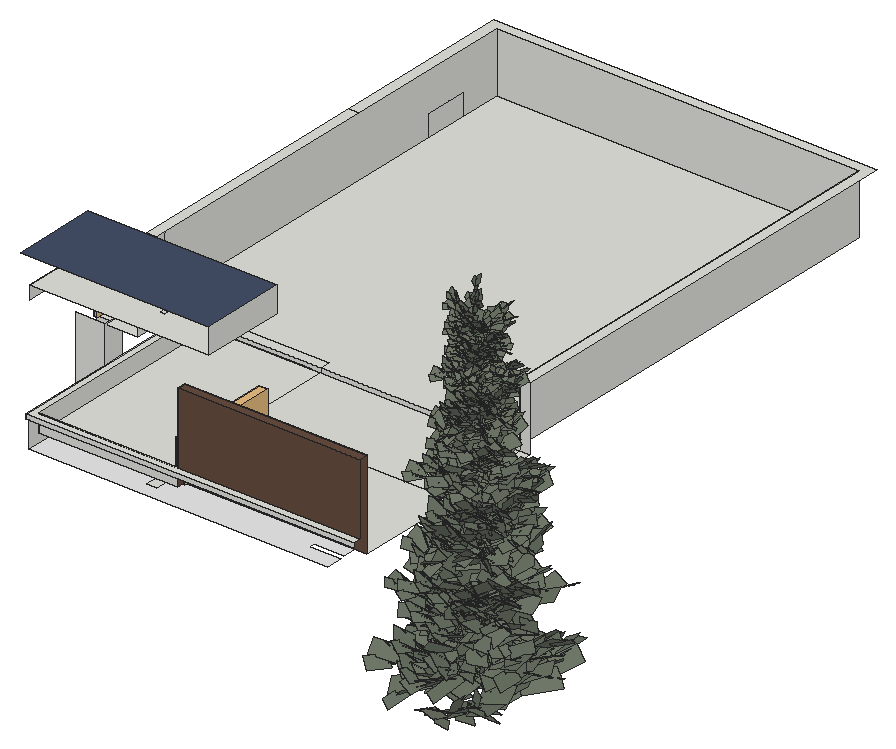
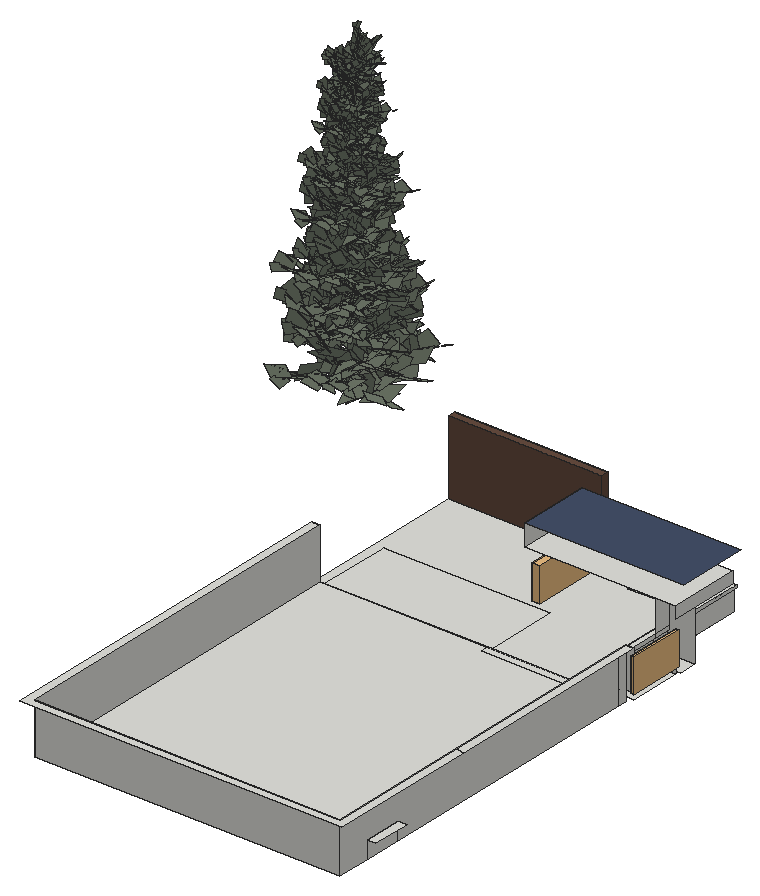
# SketchUp Ruby script. Lengths in inches.
U = 1.inch
M = Sketchup.active_model
def pt(a) = Geom::Point3d.new(a.map { |v| v * U })
def face(e, loops, mat)
  f = e.add_face(loops[0].map { |a| pt(a) })
  loops[1..].each { |l| e.add_face(l.map { |a| pt(a) }).erase! }
  f.material = f.back_material = mat if mat
  f
end
# faces: each face lists its corners as indices into pts; further lists are holes
def faces(e, pts, list, mat = nil) = list.each { |f| face(e, (f[0].is_a?(Array) ? f : [f]).map { |l| l.map { |i| pts[i] } }, mat) }
# xy, xz, yz: faces in a plane at the given z, y or x. An outline is a flat list of corners, or four numbers for a rectangle; further outlines are holes
def ring(l) = l.size == 4 ? [[l[0], l[1]], [l[2], l[1]], [l[2], l[3]], [l[0], l[3]]] : l.each_slice(2).to_a
def flat(e, list, mat, &to3) = list.each { |f| face(e, (f[0].is_a?(Array) ? f : [f]).map { |l| ring(l).map { |u, v| to3.(u, v) } }, mat) }
def xy(e, z, list, mat = nil) = flat(e, list, mat) { |x, y| [x, y, z] }
def xz(e, y, list, mat = nil) = flat(e, list, mat) { |x, z| [x, y, z] }
def yz(e, x, list, mat = nil) = flat(e, list, mat) { |y, z| [x, y, z] }
def lines(e, pts, list) = list.each { |a, b| e.add_line(pt(pts[a]), pt(pts[b])) }
# prism: a flat outline (further loops are holes) pulled along v
def prism(e, loops, v, mat = nil)
  f = face(e, loops, mat); d = Geom::Vector3d.new(v.map { |x| x * U })
  f.pushpull(f.normal.samedirection?(d) ? d.length : -d.length)
end
def box(e, o, s, mat = nil) = prism(e, [[o, [o[0] + s[0], o[1], o[2]], [o[0] + s[0], o[1] + s[1], o[2]], [o[0], o[1] + s[1], o[2]]]], [0, 0, s[2]], mat)
def at(x, y, z, deg = 0) = Geom::Transformation.translation(pt([x, y, z])) * Geom::Transformation.rotation(ORIGIN, Z_AXIS, deg.degrees)
def axes(o, x, y, z) = Geom::Transformation.new([*x, 0, *y, 0, *z, 0, *pt(o).to_a, 1])
def part(name) = M.definitions.add(name)
# library, detail: a bought-in or finely detailed component or shape, given as its bounding box
def library(name, o, s) = part(name).tap { |d| box(d.entities, o, s) }
def detail(e, o, s) = box(e.add_group.entities, o, s)
def put(e, d, t, mat = nil) = e.add_instance(d, t).tap { |i| i.material = mat if mat }
def group(e, t, mat = nil) = e.add_group.tap { |g| g.transformation = t; g.material = mat if mat }.entities
root = M.entities
M.materials.add("Marc_Shoes2").color = [68, 80, 105]
M.materials.add("Teddy_Glasses").color = [103, 77, 64]
M.materials.add("[Wood Board Cork]").color = [215, 201, 115]
M.materials.add("folha_pinheiro_fsadfaf0sa5f60a6s1d0fa19e01a601fw601").color = [111, 120, 105]
M.materials.add("white_wall").color = [233, 233, 233]
c1 = part("bough01")
p = [[11.29,3.2,8.88],[13.41,4.42,-0.24],[13.19,18.86,1.64],[11.08,17.64,10.76],[8.3,5.16,4.77],[17.24,0,0],
  [26.01,15.19,0],[17.07,20.36,4.77],[7.28,2.65,0.91],[15.18,7.21,3.36],[7.9,19.82,3.36],[0,15.26,0.91],
  [8.87,11.62,4.48],[17.62,18.34,1.72],[8.85,32.26,7.82],[0.1,25.53,10.58],[10.83,18.83,5.84],[18.73,15.63,1.77],
  [26.01,27.18,6.84],[18.11,30.37,10.91],[8.25,26.54,5.5],[14.01,28.875,8.47],[10.03,38.73,8.47],[4.26,36.4,5.5],
  [10.04,24.31,6.06],[17.58,22.66,9.11],[19.2,35.07,11.83],[11.65,36.72,8.78]]
faces(c1.entities,p,[[0,1,2,3],[4,5,6,7],[8,9,10,11],[12,13,14,15],[16,17,18,19],[20,21,22,23],[24,25,26,27]],"folha_pinheiro_fsadfaf0sa5f60a6s1d0fa19e01a601fw601")
c2 = part("Group\#64")
put(c2.entities,c1,axes([22.61,-7.4375,0.27],[0.83269,0.71876,0],[-0.71876,0.83269,0],[0,0,1.1]))
put(c2.entities,c1,axes([17.06,9.8,0.27],[1.09059,0.14358,0],[-0.14358,1.09059,0],[0,0,1.1]))
c3 = library("Group\#28",[0,0,0],[8.24,96.29,36.98])
c4 = library("Group\#29",[0,0,0],[3.15,61.52,36.98])
xy(root,239.78,[[242.31,394.5,272.99,413.5625]])
xy(root,240,[[372.21,315.12,381.21,342.06],[372.21,342.06,381.21,351.06],[372.21,351.06,381.21,359.56]])
xy(root,240,[[295.37,342.06,295.37,505.52,304.37,505.52,304.37,351.06,372.21,351.06,372.21,342.06],[381.21,342.06,549.96,351.06]],"[Wood Board Cork]")
xy(root,240,[[272.99,302.12,549.96,302.12,549.96,317.12,521.53,317.12,521.53,321.32,549.96,321.32,549.96,342.06,381.21,342.06,381.21,315.12,372.21,315.12,372.21,342.06,295.37,342.06,295.37,505.52,272.99,505.52],[304.37,351.06,372.21,351.06,372.21,359.56,381.21,359.56,381.21,351.06,549.96,351.06,549.96,505.52,304.37,505.52]],"white_wall")
xy(root,242,[[295.37,342.06,372.21,342.06,372.21,351.06,304.37,351.06,304.37,505.52,295.37,505.52],[381.21,342.06,549.96,351.06]])
xy(root,252,[[276.51,309.07,405.65,309.07,405.65,317.26,574.21,317.26,574.21,505.52,565.21,505.52,565.21,418.52,381.21,418.52,381.21,505.52,276.51,505.52],[381.21,418.52,565.21,505.52]])
xy(root,256.375,[[229.21,505.52,381.21,514.52],[381.21,505.52,565.21,505.52,565.21,898.52,229.21,898.52,229.21,514.52,381.21,514.52]])
xy(root,261.3125,[[219.74,447.9375,234.87,505.52]])
xy(root,264.16,[[558.74,302.12,564.85,305.12]])
xy(root,264.1875,[[269.99,302.12,272.99,394.5],[269.99,394.5,272.99,413.5625],[269.99,413.5625,272.99,505.52]])
xy(root,268,[[269.99,302.12,574.21,302.12,574.21,309.07,276.51,309.07,276.51,505.52,269.99,505.52],[219.74,447.9375,234.87,505.52]])
xy(root,276,[[219.74,818.95,229.21,860.95]])
xy(root,302.34,[[269.99,394.5,300.31,413.5625]])
xy(root,312,[[219.74,505.52,229.21,739.58],[565.21,505.52,574.21,505.52,574.21,907.52,219.74,907.52,219.74,739.58,229.21,739.58,229.21,898.52,565.21,898.52]])
xy(root,316.1875,[[219.74,394.5,300.31,413.5625]])
xy(root,328.22,[[219.74,369.3125,386.12,447.9375]])
xy(root,330,[[321.07,394.5,324.88,398.3125]])
xy(root,334.1875,[[405.65,309.07,574.21,317.26]],"Teddy_Glasses")
xy(root,352.25,[[211.37,369.3125,386.12,447.9375]],"Marc_Shoes2")
xz(root,302.12,[[269.99,264.1875,574.21,268]])
xz(root,309.07,[[276.51,252,405.65,268]])
xz(root,309.07,[[405.65,268,574.21,334.1875]],"Teddy_Glasses")
xz(root,317.26,[[405.65,252,574.21,334.1875]],"Teddy_Glasses")
xz(root,342.06,[[295.37,240,372.21,242],[381.21,240,549.96,242]])
xz(root,351.06,[[304.37,240,372.21,242],[381.21,240,549.96,242]])
xz(root,394.5,[[242.31,239.78,272.99,239.78,272.99,264.1875,269.99,264.1875,269.99,302.34,242.31,302.34]])
xz(root,447.9375,[[219.74,261.3125,234.87,268]])
xz(root,505.52,[[272.99,240,295.37,240,295.37,242,304.37,242,304.37,240,372.21,240,372.21,252,276.51,252,276.51,256.375,272.99,256.375],[295.37,240,304.37,242],[276.51,252,381.21,256.375],[381.21,252,565.21,256.375],[565.21,252,574.21,312],
  [229.21,256.375,229.21,261.3125,234.87,261.3125,234.87,268,269.99,268,269.99,264.1875,272.99,264.1875,272.99,256.375],[272.99,256.375,276.51,256.375,276.51,268,269.99,268,269.99,264.1875,272.99,264.1875],[229.21,261.3125,234.87,268],[219.74,268,229.21,312]])
xz(root,898.52,[[229.21,256.375,565.21,312]])
yz(root,219.74,[[369.3125,316.1875,447.9375,328.22]])
yz(root,229.21,[[505.52,256.375,514.52,312],[514.52,256.375,818.95,256.375,818.95,276,860.95,276,860.95,256.375,898.52,256.375,898.52,312,514.52,312],[818.95,256.375,860.95,276]])
yz(root,234.87,[[447.9375,261.3125,505.52,268]])
yz(root,269.99,[[302.12,264.1875,394.5,268],[394.5,264.1875,413.5625,268],[413.5625,264.1875,505.52,268],[394.5,268,413.5625,302.34]])
yz(root,272.99,[[394.5,239.78,413.5625,240],[302.12,240,394.5,264.1875],[394.5,240,413.5625,264.1875],[413.5625,240,505.52,264.1875]])
yz(root,276.51,[[309.07,252,505.52,268]])
yz(root,295.37,[[342.06,240,351.06,242],[351.06,240,505.52,242]])
yz(root,300.31,[[394.5,302.34,413.5625,316.1875]])
yz(root,304.37,[[351.06,240,505.52,242]])
yz(root,372.21,[[342.06,240,351.06,242]])
yz(root,381.21,[[342.06,240,351.06,242]])
yz(root,386.12,[[369.3125,328.22,447.9375,352.25]])
yz(root,405.65,[[309.07,252,317.26,334.1875]],"Teddy_Glasses")
yz(root,549.96,[[342.06,240,351.06,242]])
yz(root,565.21,[[505.52,256.375,898.52,312]])
p = [[558.35,302.12,264.1875],[562.09,302.12,264.1875],[562.09,306.12,264.26],[558.35,306.12,264.26]]
faces(root,p,[[0,1,2,3]])
put(root,c1,axes([793.71,158.625,286.79],[-0.73472,1.6122,0],[-1.39621,-0.63629,-1.11619],[-0.8061,-0.36736,1.93329]))
put(root,c2,axes([817.94,197.28,252.97],[-1.39482,-0.13431,0],[0.13344,-1.38585,0.15863],[-0.0152,0.1579,1.39226]))
put(root,c2,axes([736.08,217.86,253.14],[1.5292,-0.50573,0],[0.50248,1.51937,0.18233],[-0.05725,-0.17311,1.6003]))
put(root,c3,at(398.98,315.24,252))
put(root,c1,axes([763.31,217.97,252.67],[0.73472,-1.6122,0],[1.55726,0.70969,0.57778],[-0.41727,-0.19016,2.1563]))
put(root,c1,axes([783.25,194.42,252.67],[-1.65952,0.62047,0],[-0.59933,-1.60298,0.57778],[0.16059,0.42952,2.1563]))
put(root,c1,axes([754.625,192.9,252.67],[1.41278,0.77348,0],[-0.77348,1.41278,0],[0,0,2.02943]))
put(root,c2,axes([728.76,213.6,259.67],[1.39388,-0.00911,0.14345],[-0.08006,1.11225,0.84856],[-0.11938,-0.85228,1.10586]))
put(root,c2,axes([733.93,152.06,255.45],[1.31569,1.41585,0],[-1.41585,1.31569,0],[0,0,1.93279]))
put(root,c2,axes([796.66,155.73,266.49],[-0.70354,1.44888,0],[-1.44888,-0.70354,0],[0,0,2.02943]))
put(root,c4,at(218.17,445.97,268))
put(root,c1,axes([764.39,185.85,271.15],[0.62047,1.65952,0],[-1.65952,0.62047,0],[0,0,2.23237]))
put(root,c2,axes([782.14,244.15,276.91],[-0.04559,-1.39316,0.14345],[1.2949,0.01275,0.53538],[-0.53359,0.14998,1.28699]))
put(root,c2,axes([804.79,167.37,276.91],[-1.11943,0.83058,0.14345],[-0.72668,-1.07185,0.53538],[0.42707,0.3533,1.28699]))
put(root,c1,axes([770.48,218.68,307.39],[-0.17976,-1.42294,0],[-1.2323,0.15568,-0.71713],[-0.71147,0.08988,1.2421]))
put(root,c2,axes([742.41,172.19,280.73],[1.0245,1.24282,0],[-1.23483,1.01792,0.18233],[0.14069,-0.11598,1.6003]))
put(root,c2,axes([791.2,241.07,280.55],[-0.37918,-1.34899,0],[1.34032,-0.37675,0.15863],[-0.15271,0.04292,1.39226]))
put(root,c2,axes([743.74,163.83,287.26],[0.51255,1.29625,0.14345],[-1.06593,0.32757,0.84856],[0.75143,-0.41951,1.10586]))
put(root,c1,axes([760.52,213.28,308.3125],[0.93717,-1.08572,0],[0.94026,0.81161,-0.71713],[0.54286,0.46858,1.2421]))
put(root,c1,axes([771.78,167.96,321.4],[0.16997,0.69906,-1.24077],[-1.42103,0.00065,-0.1943],[-0.09414,1.25236,0.69269]))
put(root,c1,axes([754.07,194.94,299.87],[1.40596,0.28349,0],[0.27383,-1.35805,-0.37121],[0.07337,-0.36389,1.38538]))
put(root,c1,axes([771.92,192.62,289.02],[0.17921,1.29149,0],[-1.03683,0.14387,0.7774],[0.77002,-0.10685,1.04677]))
put(root,c1,axes([771.95,163.79,320.21],[0.10504,1.4304,0],[-1.23876,0.09097,-0.71713],[-0.7152,0.05252,1.2421]))
put(root,c1,axes([767.38,201.3,293.27],[0.7181,-0.49797,1.13729],[0.07809,1.32935,0.53275],[-1.23908,-0.20481,0.69269]))
put(root,c1,axes([776.33,209.38,293.27],[-0.55968,-0.67112,1.13729],[1.31719,-0.19566,0.53275],[-0.09414,1.25236,0.69269]))
put(root,c1,axes([773.43,217.75,298.29],[-0.10504,-1.4304,0],[1.38166,-0.10146,0.37121],[-0.37021,0.02719,1.38538]))
put(root,c1,axes([784.14,201.91,298.29],[-1.4304,0.10504,0],[-0.10146,-1.38166,0.37121],[0.02719,0.37021,1.38538]))
put(root,c1,axes([778.44,193.27,298.29],[-0.93717,1.08572,0],[-1.04873,-0.90524,0.37121],[0.28101,0.24256,1.38538]))
put(root,c1,axes([757.52,203.32,298.29],[1.30387,0,0],[0,1.30387,0],[0,0,1.30387]))
put(root,c1,axes([783.98,187.36,303.31],[-0.80832,0.77034,0.67325],[-0.29145,-0.99585,0.78956],[0.98069,0.33899,0.78956]))
put(root,c1,axes([787.89,215.12,329.91],[-1.08572,-0.93717,0],[0.84304,-0.97667,-0.62648],[0.40936,-0.47425,1.29019]))
put(root,c1,axes([761.63,209,307.52],[1.30387,0,0],[0,0.53448,1.18928],[0,-1.18928,0.53448]))
put(root,c1,axes([761.72,194.52,310.16],[1.08572,0.93717,0],[-0.93717,1.08572,0],[0,0,1.43425]))
put(root,c2,axes([774.95,152.49,324.26],[-0.38877,1.04178,-0.22435],[-1.02318,-0.29815,0.38858],[0.2979,0.33553,1.04185]))
put(root,c1,axes([771.92,186.51,311.59],[0.17921,1.29149,0],[-1.03683,0.14387,0.7774],[0.77002,-0.10685,1.04677]))
put(root,c1,axes([773.99,196.05,315.82],[-0.18723,1.31441,0.54255],[-1.36178,-0.32328,0.31324],[0.40936,-0.47425,1.29019]))
put(root,c2,axes([798.69,226.36,324.5],[-0.5689,-0.9814,0],[0.79296,-0.45966,0.66836],[-0.57823,0.33519,0.91655]))
put(root,c1,axes([760.2,190.11,321.91],[1.08572,0.93717,0],[0.93717,-1.08572,0],[0,0,1.43425]))
put(root,c2,axes([804.38,220.1,333.64],[-0.85129,-0.74068,0.14284],[0.72113,-0.76086,0.53309],[-0.2051,0.39907,1.28148]))
put(root,c2,axes([771.33,164.36,333.64],[-0.12433,1.12153,0.14284],[-1.03606,-0.15973,0.53309],[0.44485,-0.05857,1.28148]))
put(root,c2,axes([808.95,209.4,333.2],[-1.04232,-0.43229,0.11613],[0.44244,-0.95036,0.4334],[-0.06787,0.44353,1.04185]))
put(root,c2,axes([737.84,189.22,333.2],[1.00067,0.52149,0.11613],[-0.52358,0.90819,0.4334],[0.10627,-0.43593,1.04185]))
g1 = group(root,at(801.76,178.55,333.2))
put(g1,c1,axes([-19.16,19.03,-0.32],[-1.15379,-0.24316,0.40821],[0.34407,-1.1669,0.27742],[0.32769,0.36908,1.14604]))
put(g1,c1,axes([-21.35,-0.23,6.51],[-1.15325,0.43742,0.18888],[-0.34588,-1.1088,0.45599],[0.32769,0.36908,1.14604]))
put(root,c2,axes([732.23,199.25,330.43],[1.30387,0,0],[0,1.30387,0],[0,0,1.30387]))
put(root,c2,axes([763.4,232.93,336.29],[0.54277,-1.18552,0],[1.1779,0.53929,0.1476],[-0.1342,-0.06144,1.29548]))
g2 = group(root,at(796.3125,173.05,336.15))
put(g2,c1,axes([-13.59,23.32,-0.66],[-1.2442,0.02134,0.0923],[-0.01339,-1.24314,0.10693],[0.09378,0.10563,1.23978]))
put(g2,c1,axes([-21.78,4.61,1.56],[-1.03256,0.70035,0.01844],[-0.69429,-1.02731,0.14005],[0.09378,0.10563,1.23978]))
put(root,c2,axes([756.85,234.92,341.58],[0.76271,-0.83161,0.11613],[0.61546,0.66039,0.68693],[-0.5712,-0.39886,0.89522]))
put(root,c2,axes([807.55,213.04,337.27],[-1.00892,-0.51851,0],[0.51518,-1.00244,0.15795],[-0.0587,0.11421,1.3863]))
put(root,c2,axes([735.59,198.62,343.94],[1.05114,0.41036,0.14284],[-0.39314,0.81262,0.84492],[0.16531,-0.67678,1.10112]))
put(root,c1,axes([760.53,210.8,375.71],[0.7728,-0.92426,0],[-0.80043,-0.66926,-0.74093],[-0.46213,-0.3864,1.28334]))
put(root,c1,axes([758.15,201.59,376.66],[1.20396,-0.04415,0],[0.03823,1.04266,-0.74093],[0.02207,0.60198,1.28334]))
put(root,c1,axes([792.48,182.6,390.18],[-0.33296,0.50432,-1.28196],[-0.81295,-0.87404,-0.20075],[-0.82445,0.65818,0.71569]))
put(root,c1,axes([765.75,187.13,367.93],[0.62949,1.02724,0],[0.99223,-0.60804,-0.38354],[0.26587,-0.16292,1.43138]))
put(root,c2,axes([759.95,162.77,352.76],[0.47151,1.21562,0],[-1.21562,0.47151,0],[0,0,1.30387]))
put(root,c1,axes([777.39,196.79,356.72],[-0.69223,0.84876,0],[-0.6814,-0.55573,0.80321],[0.50605,0.41272,1.08152]))
put(root,c2,axes([739.8125,204.01,358.62],[1.30157,0.07733,0],[-0.07683,1.2932,0.1476],[0.00875,-0.14734,1.29548]))
put(root,c1,axes([795.14,180.33,388.95],[-0.82011,0.88255,0],[-0.76431,-0.71024,-0.74093],[-0.44127,-0.41006,1.28334]))
put(root,c1,axes([769.59,209.08,361.11],[0.09294,-0.72814,1.17505],[0.87357,0.69863,0.55043],[-0.82445,0.65818,0.71569]))
put(root,c1,axes([769.45,198.96,361.11],[0.71703,0.15713,1.17505],[-0.77334,0.80818,0.55043],[-0.58248,-0.87956,0.71569]))
put(root,c1,axes([762.79,212.09,366.3],[0.82011,-0.88255,0],[0.85247,0.79217,0.38354],[-0.22842,-0.21226,1.43138]))
put(root,c1,axes([780.71,201.17,366.3],[-1.20396,0.04415,0],[-0.04264,-1.16294,0.38354],[0.01143,0.31161,1.43138]))
put(root,c1,axes([778.66,209.62,366.3],[-0.88255,-0.82011,0],[0.79217,-0.85247,0.38354],[-0.21226,0.22842,1.43138]))
put(root,c1,axes([762.57,194.05,366.3],[0.74556,0.80232,0],[-0.80232,0.74556,0],[0,0,1.34715]))
put(root,c1,axes([787.52,201.2,371.49],[-0.93622,-0.0569,0.6956],[0.44613,-0.74877,0.81577],[0.35217,0.79729,0.81577]))
put(root,c1,axes([772.68,219.48,398.97],[-0.04415,-1.20396,0],[1.08303,-0.03971,-0.64728],[0.52589,-0.01928,1.33303]))
put(root,c1,axes([761.43,199.82,375.84],[0.74556,0.80232,0],[-0.32889,0.30562,1.22877],[0.73181,-0.68004,0.55223]))
put(root,c1,axes([770.38,191.6,378.57],[0.04415,1.20396,0],[-1.20396,0.04415,0],[0,0,1.48187]))
put(root,c2,axes([803.8125,175.71,393.13],[-0.86335,0.35647,-0.23179],[-0.4016,-0.80008,0.40148],[-0.03612,0.37517,1.07644]))
put(root,c1,axes([781.15,193.29,380.04],[-0.69223,0.84876,0],[-0.6814,-0.55573,0.80321],[0.50605,0.41272,1.08152]))
put(root,c1,axes([776.46,200.03,384.41],[-0.91586,0.63637,0.56056],[-0.57975,-1.02281,0.32364],[0.52589,-0.01928,1.33303]))
put(root,c2,axes([771.93,232.55,393.38],[0.27859,-0.91123,0],[0.73626,0.2251,0.69055],[-0.53689,-0.16414,0.94698]))
put(root,c1,axes([772.23,188.14,390.71],[0.04415,1.20396,0],[1.20396,-0.04415,0],[0,0,1.48187]))
put(root,c2,axes([803.1,207.11,402.375],[-0.89445,-0.31368,0.11999],[0.32651,-0.81781,0.44779],[-0.03612,0.37517,1.07644]))
put(root,c2,axes([788.24,229.17,402.375],[-0.33,-0.88856,0.11999],[0.83778,-0.27117,0.44779],[-0.31173,0.21185,1.07644]))
put(root,c2,axes([750.62,176.16,399.51],[0.74556,0.80232,0],[-0.80232,0.74556,0],[0,0,1.34715]))
put(root,c2,axes([803.38,200.61,405.42],[-0.94848,-0.09133,0],[0.09074,-0.94238,0.13268],[-0.01034,0.10737,1.16449]))
put(root,c2,axes([747.71,214.6,405.5625],[1.03986,-0.3439,0],[0.34169,1.03317,0.1525],[-0.03893,-0.11771,1.33849]))
put(root,c2,axes([759.99,173.87,411.41],[0.2513,0.91394,0.09755],[-0.85823,0.19713,0.36406],[0.32901,-0.18387,0.87516]))
put(root,c2,axes([742.74,211.71,418.44],[0.94784,-0.00619,0.09755],[-0.05444,0.75633,0.57702],[-0.08118,-0.57955,0.75199]))
put(root,c2,axes([779.04,232.48,430.16],[-0.031,-0.94735,0.09755],[0.88053,0.00867,0.36406],[-0.36284,0.10199,0.87516]))
put(root,c2,axes([794.43,180.27,430.16],[-0.76121,0.5648,0.09755],[-0.49414,-0.72886,0.36406],[0.29041,0.24025,0.87516]))
put(root,c2,axes([785.2,230.39,428.49],[-0.25785,-0.91732,0],[0.91142,-0.25619,0.13268],[-0.10384,0.02919,1.16449]))
put(root,c2,axes([788.91,172.35,427.84],[-0.47841,0.98524,0],[-0.98524,-0.47841,0],[0,0,1.09525]))
put(root,c2,axes([752.02,183.55,432.76],[0.69666,0.84512,0],[-0.83969,0.69218,0.12399],[0.09567,-0.07886,1.08821]))
put(root,c2,axes([752.92,177.86,437.2],[0.34854,0.88145,0.09755],[-0.72483,0.22275,0.57702],[0.51097,-0.28527,0.75199]))
put(root,c2,axes([769.63,179.43,446.69],[-0.08205,0.74021,0.10041],[-0.6838,-0.10542,0.37472],[0.2936,-0.03865,0.90078]))
put(root,c2,axes([791.45,216.22,446.69],[-0.56185,-0.48885,0.10041],[0.47595,-0.50217,0.37472],[-0.13536,0.26339,0.90078]))
put(root,c2,axes([762.12,178.375,444.3],[0.3112,0.80231,0],[-0.80231,0.3112,0],[0,0,1.12732]))
put(root,c2,axes([748.83,205.6,449.36],[0.85904,0.05104,0],[-0.05071,0.85351,0.12762],[0.00578,-0.09725,1.12008]))
put(root,c2,axes([793.54,211.55,449.24],[-0.66589,-0.34222,0],[0.34002,-0.66161,0.11103],[-0.03874,0.07538,0.97447]))
put(root,c2,axes([746.04,202.04,453.93],[0.69375,0.27084,0.10041],[-0.25947,0.53633,0.59392],[0.1091,-0.44667,0.77401]))
put(root,c1,axes([762.51,210.08,476.26],[0.51005,-0.61001,0],[-0.52828,-0.44171,-0.52082],[-0.30501,-0.25502,0.90209]))
put(root,c1,axes([760.9375,204,476.93],[0.79462,-0.02914,0],[0.02523,0.68816,-0.52082],[0.01457,0.39731,0.90209]))
put(root,c1,axes([783.59,191.47,486.4375],[-0.21976,0.33285,-0.90113],[-0.53655,-0.57687,-0.14111],[-0.54414,0.4344,0.50308]))
put(root,c1,axes([765.95,194.46,470.79],[0.41546,0.67798,0],[0.65487,-0.40131,-0.2696],[0.17547,-0.10753,1.00615]))
put(root,c1,axes([773.63,200.83,462.91],[-0.45687,0.56018,0],[-0.44972,-0.36678,0.5646],[0.33399,0.2724,0.76023]))
put(root,c1,axes([785.35,189.96,485.57],[-0.54127,0.58248,0],[-0.50444,-0.46876,-0.52082],[-0.29124,-0.27064,0.90209]))
put(root,c1,axes([768.39,202.26,466],[0.47324,0.10371,0.82598],[-0.5104,0.5334,0.38692],[-0.38444,-0.58051,0.50308]))
put(root,c1,axes([768.49,208.94,466],[0.06134,-0.48057,0.82598],[0.57656,0.4611,0.38692],[-0.54414,0.4344,0.50308]))
put(root,c1,axes([774.47,209.3,469.65],[-0.58248,-0.54127,0],[0.52283,-0.56263,0.2696],[-0.14009,0.15076,1.00615]))
put(root,c1,axes([775.83,203.72,469.65],[-0.79462,0.02914,0],[-0.02814,-0.76754,0.2696],[0.00754,0.20566,1.00615]))
put(root,c1,axes([763.99,210.93,469.65],[0.54127,-0.58248,0],[0.56263,0.52283,0.2696],[-0.15076,-0.14009,1.00615]))
put(root,c1,axes([763.85,199.02,469.65],[0.49207,0.52953,0],[-0.52953,0.49207,0],[0,0,0.94695]))
put(root,c1,axes([780.32,203.74,473.29],[-0.61791,-0.03755,0.48895],[0.29445,-0.49419,0.57343],[0.23243,0.52621,0.57343]))
put(root,c1,axes([770.52,215.81,492.61],[-0.02914,-0.79462,0],[0.7148,-0.02621,-0.45499],[0.34709,-0.01273,0.93702]))
put(root,c1,axes([763.1,202.83,476.35],[0.49207,0.52953,0],[-0.21707,0.20171,0.86373],[0.48299,-0.44883,0.38818]))
put(root,c1,axes([769.01,197.4,478.27],[0.02914,0.79462,0],[-0.79462,0.02914,0],[0,0,1.04165]))
put(root,c2,axes([791.07,186.92,488.51],[-0.56981,0.23527,-0.16293],[-0.26505,-0.52805,0.28221],[-0.02384,0.24761,0.75666]))
put(root,c1,axes([776.11,198.52,479.31],[-0.45687,0.56018,0],[-0.44972,-0.36678,0.5646],[0.33399,0.2724,0.76023]))
put(root,c1,axes([773.02,202.97,482.38],[-0.60447,0.42001,0.39404],[-0.38263,-0.67505,0.2275],[0.34709,-0.01273,0.93702]))
put(root,c2,axes([770.03,224.44,488.68],[0.18387,-0.60141,0],[0.48593,0.14856,0.48541],[-0.35435,-0.10834,0.66566]))
put(root,c1,axes([770.23,195.12,486.8],[0.02914,0.79462,0],[0.79462,-0.02914,0],[0,0,1.04165]))
put(root,c2,axes([780.79,222.2,495],[-0.2178,-0.58645,0.08434],[0.55294,-0.17898,0.31477],[-0.20574,0.13982,0.75666]))
put(root,c2,axes([762.15,185.7,495],[0.16586,0.6032,0.08434],[-0.56643,0.1301,0.31477],[0.21714,-0.12136,0.75666]))
put(root,c2,axes([790.6,207.64,495],[-0.59034,-0.20703,0.08434],[0.21549,-0.53975,0.31477],[-0.02384,0.24761,0.75666]))
put(root,c2,axes([755.96,187.21,492.99],[0.49207,0.52953,0],[-0.52953,0.49207,0],[0,0,0.94695]))
put(root,c2,axes([790.79,203.35,497.14],[-0.626,-0.06028,0],[0.05989,-0.62197,0.09326],[-0.00682,0.07086,0.81855]))
put(root,c2,axes([754.04,212.59,497.25],[0.6863,-0.22697,0],[0.22551,0.68189,0.1072],[-0.02569,-0.07769,0.94086]))
put(root,c2,axes([750.76,210.68,501.09],[0.62557,-0.00409,0.08434],[-0.03593,0.49918,0.49889],[-0.05358,-0.3825,0.65017]))
put(root,c2,axes([774.72,224.39,511.22],[-0.02046,-0.62525,0.08434],[0.58115,0.00572,0.31477],[-0.23947,0.06731,0.75666]))
put(root,c2,axes([784.88,189.93,511.22],[-0.5024,0.37277,0.08434],[-0.32613,-0.48105,0.31477],[0.19167,0.15856,0.75666]))
put(root,c2,axes([781.24,184.7,509.21],[-0.31575,0.65026,0],[-0.65026,-0.31575,0],[0,0,0.94695]))
put(root,c2,axes([756.89,192.09,513.46],[0.4598,0.55778,0],[-0.55419,0.45684,0.1072],[0.06314,-0.05205,0.94086]))
put(root,c2,axes([778.78,223.01,513.36],[-0.17018,-0.60543,0],[0.60154,-0.16908,0.09326],[-0.06854,0.01926,0.81855]))
put(root,c2,axes([757.48,188.34,517.3],[0.23003,0.58176,0.08434],[-0.47839,0.14701,0.49889],[0.33724,-0.18828,0.65017]))
put(root,c1,axes([763.6875,200.48,531.27],[0.60821,-0.07037,0],[-0.06094,-0.52672,-0.40103],[-0.03519,-0.3041,0.69461]))
put(root,c1,axes([766.04,196.25,531.79],[0.45927,0.4049,0],[-0.35065,0.39774,-0.40103],[-0.20245,0.22963,0.69461]))
put(root,c1,axes([785.33,201.26,539.11],[-0.29916,0.06943,-0.69387],[0.00607,-0.60659,-0.10866],[-0.53417,-0.04578,0.38737]))
put(root,c1,axes([773.89,193.58,527.0625],[-0.1273,0.59889,0],[0.57848,0.12296,-0.20759],[0.155,0.03295,0.77474]))
put(root,c1,axes([774.81,201.21,521],[-0.55209,0.07072,0],[-0.05678,-0.44323,0.43474],[0.04217,0.32917,0.58538]))
put(root,c1,axes([787.11,201.35,538.44],[-0.61106,0.03844,0],[-0.03329,-0.52919,-0.40103],[-0.01922,-0.30553,0.69461]))
put(root,c1,axes([771.12,199.23,523.375],[0.20935,0.30876,0.636],[-0.5678,0.02739,0.29792],[0.09297,-0.528,0.38737]))
put(root,c1,axes([767.63,203.02,523.375],[0.28898,-0.23591,0.636],[0.07763,0.56313,0.29792],[-0.53417,-0.04578,0.38737]))
put(root,c1,axes([764.07,201.74,526.18],[0.61106,-0.03844,0],[0.03713,0.59024,0.20759],[-0.00995,-0.15815,0.77474]))
put(root,c1,axes([770.79,206.39,526.18],[-0.03844,-0.61106,0],[0.59024,-0.03713,0.20759],[-0.15815,0.00995,0.77474]))
put(root,c1,axes([774.5,203.99,526.18],[-0.45927,-0.4049,0],[0.3911,-0.44362,0.20759],[-0.1048,0.11887,0.77474]))
put(root,c1,axes([770.3,195.02,526.18],[-0.00583,0.55657,0],[-0.55657,-0.00583,0],[0,0,0.72915]))
put(root,c1,axes([777,206.38,528.99],[-0.32522,-0.34849,0.37649],[0.4264,-0.11996,0.44154],[-0.14909,0.41711,0.44154]))
put(root,c1,axes([765.13,207.93,543.86],[0.4049,-0.45927,0],[0.41314,0.36423,-0.35034],[0.20061,0.17686,0.72151]))
put(root,c1,axes([767.86,196.75,531.34],[-0.00583,0.55657,0],[-0.22815,-0.00239,0.66507],[0.50766,0.00532,0.2989]))
put(root,c1,axes([774.04,196.85,532.82],[-0.4049,0.45927,0],[-0.45927,-0.4049,0],[0,0,0.80207]))
put(root,c2,axes([791.92,202.68,540.71],[-0.44296,-0.17061,-0.12546],[0.13184,-0.43543,0.2173],[-0.14456,0.12566,0.58263]))
put(root,c1,axes([777.41,201.24,533.62],[-0.55209,0.07072,0],[-0.05678,-0.44323,0.43474],[0.04217,0.32917,0.58538]))
put(root,c1,axes([773.33,202.08,535.98],[-0.56024,-0.0858,0.30341],[0.14408,-0.57985,0.17517],[0.20061,0.17686,0.72151]))
put(root,c2,axes([760.28,212.49,540.84],[0.42147,-0.23845,0],[0.19267,0.34054,0.37376],[-0.1405,-0.24833,0.51256]))
put(root,c1,axes([775.93,196.22,539.39],[-0.4049,0.45927,0],[0.45927,0.4049,0],[0,0,0.80207]))
put(root,c2,axes([767.48,216.94,545.71],[0.18919,-0.443,0.06494],[0.4037,0.19311,0.24237],[-0.18902,-0.03095,0.58263]))
put(root,c2,axes([776.41,186.68,545.71],[-0.22708,0.42482,0.06494],[-0.38533,-0.22756,0.24237],[0.18561,0.04731,0.58263]))
put(root,c2,axes([780.68,214.01,545.71],[-0.21999,-0.42853,0.06494],[0.40645,-0.18725,0.24237],[-0.14456,0.12566,0.58263]))
put(root,c2,axes([772.15,184.24,544.16],[-0.00583,0.55657,0],[-0.55657,-0.00583,0],[0,0,0.72915]))
put(root,c2,axes([783.05,211.71,547.35],[-0.31769,-0.36547,0],[0.36312,-0.31565,0.07181],[-0.04137,0.03596,0.63028]))
put(root,c2,axes([757.63,197.4,547.43],[0.50363,0.23699,0],[-0.23547,0.50039,0.08254],[0.02683,-0.05701,0.72446]))
put(root,c2,axes([756.8125,194.59,550.39],[0.35157,0.32929,0.06494],[-0.28465,0.25976,0.38415],[0.17281,-0.24204,0.50063]))
put(root,c2,axes([762.93,214.95,558.19],[0.31998,-0.36007,0.06494],[0.32156,0.31123,0.24237],[-0.16943,-0.08933,0.58263]))
put(root,c2,axes([786.87,201.08,558.19],[-0.47819,-0.05808,0.06494],[0.07281,-0.44154,0.24237],[0.02301,0.19015,0.58263]))
put(root,c2,axes([787.6,196.23,556.64],[-0.52101,0.19584,0],[-0.19584,-0.52101,0],[0,0,0.72915]))
put(root,c2,axes([770.09,187.46,559.92],[-0.03883,0.55525,0],[-0.55168,-0.03858,0.08254],[0.06286,0.0044,0.72446]))
put(root,c2,axes([765.93,216.33,559.84],[0.22585,-0.42835,0],[0.4256,0.22439,0.07181],[-0.04849,-0.02557,0.63028]))
put(root,c2,axes([772.41,185.67,562.875],[-0.17987,0.44686,0.06494],[-0.34512,-0.17145,0.38415],[0.28815,0.07359,0.50063]))
put(root,c2,axes([772.9375,188.56,572.01],[-0.163,0.45738,0.02212],[-0.0867,-0.03406,0.53609],[0.49307,0.1937,0.24175]))
